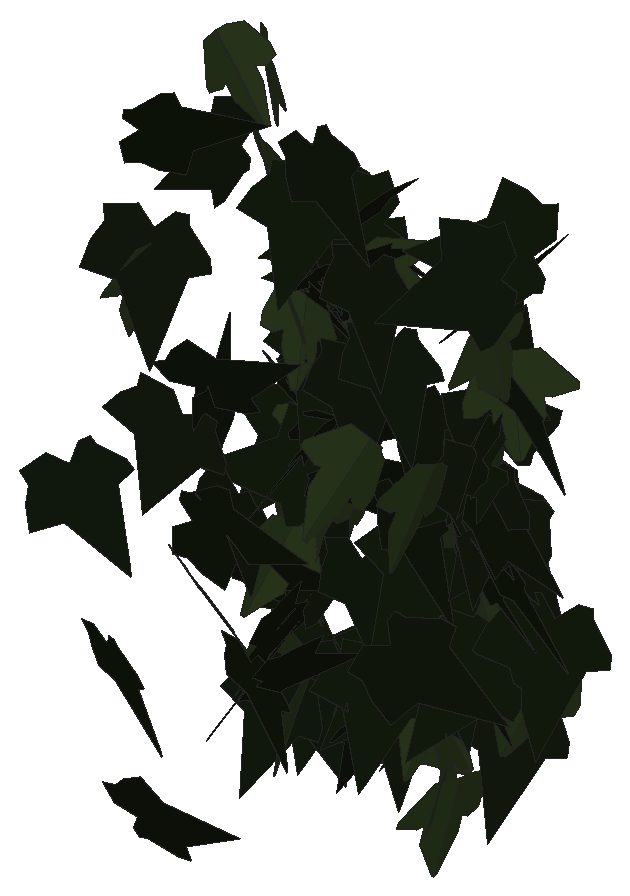
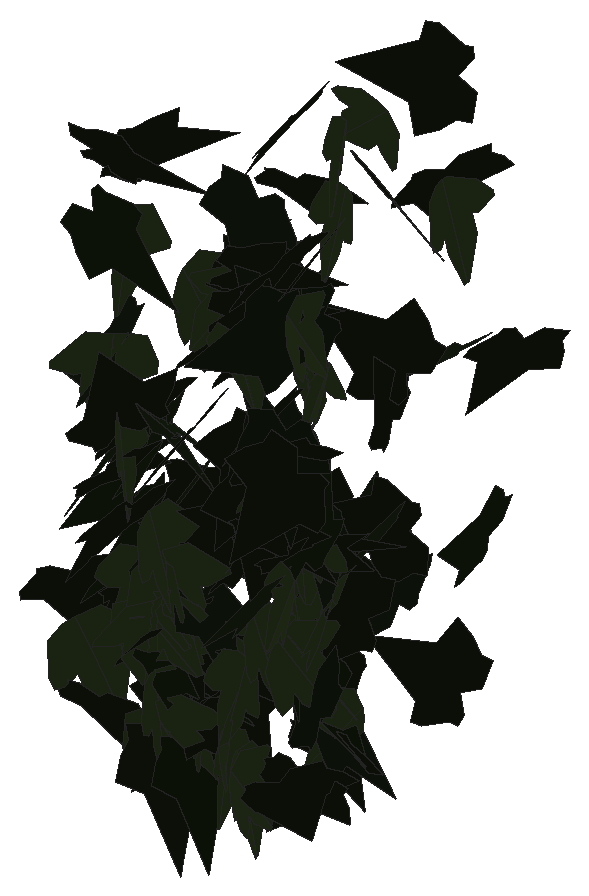
# SketchUp Ruby script. Lengths in inches.
U = 1.inch
M = Sketchup.active_model
def pt(a) = Geom::Point3d.new(a.map { |v| v * U })
def face(e, loops, mat)
  f = e.add_face(loops[0].map { |a| pt(a) })
  loops[1..].each { |l| e.add_face(l.map { |a| pt(a) }).erase! }
  f.material = f.back_material = mat if mat
  f
end
# faces: each face lists its corners as indices into pts; further lists are holes
def faces(e, pts, list, mat = nil) = list.each { |f| face(e, (f[0].is_a?(Array) ? f : [f]).map { |l| l.map { |i| pts[i] } }, mat) }
# xy, xz, yz: faces in a plane at the given z, y or x. An outline is a flat list of corners, or four numbers for a rectangle; further outlines are holes
def ring(l) = l.size == 4 ? [[l[0], l[1]], [l[2], l[1]], [l[2], l[3]], [l[0], l[3]]] : l.each_slice(2).to_a
def flat(e, list, mat, &to3) = list.each { |f| face(e, (f[0].is_a?(Array) ? f : [f]).map { |l| ring(l).map { |u, v| to3.(u, v) } }, mat) }
def xy(e, z, list, mat = nil) = flat(e, list, mat) { |x, y| [x, y, z] }
def xz(e, y, list, mat = nil) = flat(e, list, mat) { |x, z| [x, y, z] }
def yz(e, x, list, mat = nil) = flat(e, list, mat) { |y, z| [x, y, z] }
def lines(e, pts, list) = list.each { |a, b| e.add_line(pt(pts[a]), pt(pts[b])) }
# prism: a flat outline (further loops are holes) pulled along v
def prism(e, loops, v, mat = nil)
  f = face(e, loops, mat); d = Geom::Vector3d.new(v.map { |x| x * U })
  f.pushpull(f.normal.samedirection?(d) ? d.length : -d.length)
end
def box(e, o, s, mat = nil) = prism(e, [[o, [o[0] + s[0], o[1], o[2]], [o[0] + s[0], o[1] + s[1], o[2]], [o[0], o[1] + s[1], o[2]]]], [0, 0, s[2]], mat)
def at(x, y, z, deg = 0) = Geom::Transformation.translation(pt([x, y, z])) * Geom::Transformation.rotation(ORIGIN, Z_AXIS, deg.degrees)
def axes(o, x, y, z) = Geom::Transformation.new([*x, 0, *y, 0, *z, 0, *pt(o).to_a, 1])
def part(name) = M.definitions.add(name)
# library, detail: a bought-in or finely detailed component or shape, given as its bounding box
def library(name, o, s) = part(name).tap { |d| box(d.entities, o, s) }
def detail(e, o, s) = box(e.add_group.entities, o, s)
def put(e, d, t, mat = nil) = e.add_instance(d, t).tap { |i| i.material = mat if mat }
def group(e, t, mat = nil) = e.add_group.tap { |g| g.transformation = t; g.material = mat if mat }.entities
root = M.entities
M.materials.add("efeu1").color = [18, 25, 13]
M.materials.add("efeu2").color = [43, 57, 29]
c1 = part("ivyleaf_9")
p = [[1.54,2.16,1.25],[1.36,2.04,1.19],[-0.21,0.99,0.68],[-0.71,1.11,0.82],[-0.85,0.86,0.67],[-0.8,0.17,0.21],
  [-0.9,-0.01,0.1],[-0.67,-0.16,-0.02],[-0.08,-0.08,-0.05],[-0.03,-0.6,-0.4],[0.65,-0.88,-0.66],[0.83,-0.6,-0.49],
  [1.29,-0.42,-0.43],[1.8125,-0.07,-0.26],[1.21,0.44,0.15]]
faces(c1.entities,p,[[0,1,2,3,4,5,6,7,8,9,10,11,12,13,14]],"efeu1")
c2 = part("ivyleaf_10")
p = [[0,0.5,-0.03],[-0.0625,2.02,-0.43],[-0.19,2.01,-0.46],[-0.54,1.05,-0.29],[-0.52,0.625,-0.18],[-0.83,0.76,-0.28],
  [-1.16,0.64,-0.33],[-1.15,0.33,-0.24],[-0.77,-0.39,0.02],[-0.3,-0.51,0.16],[0.04,-0.48,0.23],[-0.02,2.01,-0.4375],
  [-0.06,2.01,-0.43],[0.04,-0.49,0.23],[0.67,-0.49,0.14],[1.38,0.36,-0.2],[1.375,0.51,-0.24],[0.81,0.65,-0.19],
  [0.62,0.59,-0.15],[0.6,1.09,-0.28],[0.5,1.23,-0.31]]
faces(c2.entities,p,[[0,1,2,3,4,5,6,7,8,9,10],[11,12,0,13,14,15,16,17,18,19,20]],"efeu2")
put(root,c1,axes([7.24,223.58,236.84],[0.37427,-0.2409,-0.10953],[0.09006,-0.06455,0.43891],[-0.2693,-0.3564,-0.00546]))
put(root,c2,axes([7.36,223.84,236.4375],[-0.32136,0.30247,-0.09976],[0.06352,-0.07665,-0.4411],[-0.33676,-0.30309,0.01199]))
put(root,c1,axes([7.35,223.68,237.92],[0.27793,0.32979,0.12409],[0.06108,0.10703,-0.43453],[-0.37381,0.26269,0.02126]))
put(root,c1,axes([7.12,223.52,234.79],[0.11111,-0.2186,0.37621],[0.18138,-0.3205,-0.25111],[0.41889,0.19676,0.00894]))
put(root,c1,axes([7.56,222.75,234.28],[-0.29523,0.23042,-0.25771],[0.14245,-0.2208,-0.36485],[-0.33654,-0.29559,0.07165]))
put(root,c2,axes([7.39,223.09,235.83],[-0.18841,0.3982,-0.0157],[0.00906,-0.01281,-0.45212],[-0.43027,-0.17464,-0.00264]))
put(root,c2,axes([7.46,222.55,234.17],[0.05435,0.1028,0.43646],[-0.12157,0.41104,-0.09067],[-0.45053,-0.09851,0.07712]))
put(root,c1,axes([7.55,223.45,236.71],[-0.32967,-0.3444,0.15068],[-0.05475,-0.1543,-0.47244],[0.37191,-0.328,0.06403]))
put(root,c1,axes([7.44,223.79,233.88],[-0.23188,-0.43865,-0.06175],[0.01831,0.06015,-0.49603],[0.4426,-0.2323,-0.01183]))
put(root,c2,axes([7.55,223.49,235.4],[-0.01446,-0.42559,0.26203],[-0.01458,-0.26167,-0.42581],[0.49958,-0.01995,-0.00484]))
put(root,c1,axes([7.8,221.77,240.93],[-0.40723,0.20452,0.07511],[-0.06788,0.03559,-0.44612],[-0.2242,-0.38227,-0.00135]))
put(root,c1,axes([7.36,219.5,237.84],[0.015,-0.31293,-0.31392],[0.03892,0.30179,-0.32366],[0.46794,-0.01507,0.03698]))
put(root,c2,axes([7.59,220.52,240.05],[0.03065,-0.49801,0.0324],[0.00164,-0.03236,-0.49895],[0.49906,0.0307,-0.00035]))
put(root,c1,axes([7.73,223.78,237.16],[-0.43087,-0.17183,0.02401],[-0.02319,-0.00852,-0.45176],[0.1858,-0.39953,-0.0007]))
put(root,c2,axes([7.68,222.45,241.68],[-0.32271,0.29985,0.10416],[-0.10724,0.04183,-0.4383],[-0.32415,-0.31235,0.0413]))
put(root,c1,axes([7.41,221.6875,235.39],[0.38957,-0.18257,-0.16698],[0.15944,-0.06377,0.42035],[-0.20862,-0.38965,0.00945]))
put(root,c1,axes([7.8,222.75,234.79],[-0.23411,0.322,-0.20421],[0.08926,-0.18042,-0.40258],[-0.39741,-0.2302,0.02988]))
put(root,c2,axes([7.61,223.28,239.59],[0.12695,-0.35049,0.23844],[0.08191,-0.21638,-0.38445],[0.44484,0.13987,0.00274]))
put(root,c1,axes([7.78,223.3,238.13],[0.00225,0.43462,-0.01872],[-0.00118,-0.018,-0.45201],[-0.46979,0.00212,0.00104]))
put(root,c1,axes([7.43,222.25,236.3],[0.0694,-0.39192,0.18456],[0.0824,-0.1662,-0.41048],[0.45728,0.08943,0.04596]))
put(root,c1,axes([8.01,222.94,236.51],[-0.3298,0.04514,0.31875],[-0.3287,-0.124,-0.29639],[0.06241,-0.4145,0.12338]))
put(root,c2,axes([7.6,223.21,236.81],[0.46694,0.03975,0.02779],[0.02546,0.03467,-0.45029],[-0.04503,0.43179,0.0336]))
put(root,c1,axes([7.74,222.7,233.91],[-0.42643,-0.11545,-0.14708],[0.14318,0.05035,-0.42769],[0.13555,-0.41637,-0.01094]))
put(root,c2,axes([7.47,222.06,241.88],[-0.32691,-0.00389,-0.32488],[0.29934,-0.20406,-0.27666],[-0.15569,-0.38415,0.15025]))
put(root,c1,axes([7.5,223.36,233.78],[-0.1878,-0.22057,-0.34546],[0.28115,0.21169,-0.28792],[0.32619,-0.30945,0.04927]))
put(root,c1,axes([7.75,221.4,237.55],[-0.00302,-0.21042,0.39594],[0.15023,0.36029,0.20816],[-0.44512,0.12303,0.06757]))
put(root,c1,axes([7.91,222.47,236.67],[-0.07128,0.40881,0.13852],[-0.01709,0.13235,-0.43064],[-0.46405,-0.06767,-0.00542]))
put(root,c1,axes([7.48,220,235.46],[0.27283,-0.33635,0.11522],[0.06414,-0.09393,-0.43739],[0.37704,0.25936,-0.00897]))
put(root,c2,axes([7.8,223.71,235.7],[0.03527,-0.42599,0.08507],[0.01902,-0.08066,-0.44418],[0.46809,0.03538,0.01164]))
put(root,c1,axes([7.4,221.59,236.27],[0.20707,0.03161,-0.40475],[0.31781,0.27329,0.17385],[0.27718,-0.33696,0.10303]))
put(root,c1,axes([7.68,220.49,240.39],[-0.11012,-0.47615,-0.10561],[0.013,0.10537,-0.4886],[0.48755,-0.11035,-0.01082]))
put(root,c1,axes([8.09,223,235.34],[-0.398,0.2145,0.08953],[-0.08088,0.04246,-0.44345],[-0.23615,-0.37605,0.001]))
put(root,c2,axes([7.75,222.72,238.62],[-0.29857,0.33089,-0.05983],[0.03775,-0.04576,-0.44842],[-0.36075,-0.27865,0.00259]))
put(root,c2,axes([7.83,222.57,235.77],[0.1551,0.30588,-0.28489],[-0.13785,-0.24257,-0.35129],[-0.42149,0.19189,0.01006]))
put(root,c1,axes([7.4,222.35,235.47],[0.25502,-0.08858,0.36861],[0.37425,-0.07933,-0.26073],[0.12494,0.41843,0.0286]))
put(root,c2,axes([7.87,222.23,240.65],[-0.39979,0.22056,0.06194],[-0.05517,0.03062,-0.44814],[-0.24049,-0.37369,-0.00016]))
put(root,c1,axes([7.58,223.86,236.39],[0.3108,-0.31463,-0.08959],[-0.00923,0.10757,-0.43826],[0.35218,0.28047,0.06758]))
put(root,c2,axes([7.79,223.53,237.76],[-0.04218,0.42973,-0.05723],[-0.00017,-0.05527,-0.44873],[-0.4679,-0.03872,0.00532]))
put(root,c1,axes([7.84,223.48,237.88],[-0.24948,-0.36844,-0.01136],[0.00513,0.00991,-0.45226],[0.39805,-0.23104,-0.00129]))
put(root,c1,axes([7.72,220.89,237.97],[-0.18046,-0.42997,0.18045],[0.11887,-0.22952,-0.42801],[0.45089,-0.11157,0.18506]))
put(root,c2,axes([7.86,223.99,233.84],[0.11769,-0.34318,0.25385],[0.08691,-0.23051,-0.37442],[0.44644,0.13535,0.00597]))
put(root,c1,axes([7.9,222.03,234.78],[0.0902,0.24019,0.36705],[0.15191,0.32406,-0.26398],[-0.43532,0.16285,-0.01606]))
put(root,c1,axes([7.625,220.43,241.65],[0.17402,0.2237,-0.34995],[0.15382,0.30756,0.28357],[0.40837,-0.21117,0.04231]))
put(root,c2,axes([8.06,222.93,236.18],[0.25243,-0.3119,-0.20089],[-0.10324,0.16935,-0.40468],[0.38253,0.25152,0.02336]))
put(root,c2,axes([8.02,223.75,233.82],[0.12082,-0.48391,-0.03513],[-0.00062,0.03605,-0.4987],[0.48518,0.12055,0.00811]))
put(root,c2,axes([7.79,224.4,234.52],[0.06042,-0.17406,0.4105],[0.31712,-0.27622,-0.16996],[0.34131,0.28746,0.08525]))
put(root,c1,axes([7.66,221.31,238.17],[0.0865,-0.13267,0.42272],[0.45455,-0.0484,-0.10267],[0.08136,0.41144,0.12423]))
put(root,c1,axes([7.78,223.3125,239.43],[0.42696,-0.07853,0.17015],[0.17861,-0.00561,-0.41839],[0.08071,0.42782,0.02575]))
put(root,c1,axes([8.16,223.08,237.15],[0.27483,0.33066,-0.12793],[-0.07628,-0.10085,-0.4339],[-0.37331,0.26404,-0.00552]))
put(root,c2,axes([8.13,222.39,234.06],[0.20988,-0.37631,0.10321],[0.03954,-0.09276,-0.44035],[0.41845,0.19751,-0.01016]))
put(root,c2,axes([8.04,222.5625,238.71],[0.45478,-0.08414,0.07227],[0.0747,-0.00851,-0.44656],[0.09117,0.4267,0.00535]))
put(root,c1,axes([7.77,220.18,233.43],[0.17525,-0.12796,0.39809],[0.38661,-0.14492,-0.2082],[0.20133,0.38968,0.0533]))
put(root,c1,axes([8,222.46,240.06],[0.22938,-0.36692,-0.10129],[-0.04876,0.08639,-0.4409],[0.40709,0.2171,0.00426]))
put(root,c1,axes([8,222.38,239.22],[0.45822,-0.09587,-0.00494],[-0.00477,0.00201,-0.45237],[0.10356,0.4243,0.00102]))
put(root,c1,axes([8.15,223.06,240.07],[-0.01314,-0.4924,0.08583],[0.01297,-0.08617,-0.49235],[0.49966,-0.01071,0.01504]))
put(root,c2,axes([8.34,223.46,234.86],[-0.43023,0.17463,0.00638],[-0.00592,0.00278,-0.45235],[-0.18863,-0.3984,-0.00036]))
put(root,c2,axes([8.38,223.54,233.92],[0.04319,-0.38271,-0.21099],[0.02045,0.20509,-0.39848],[0.46736,0.0264,0.03693]))
put(root,c1,axes([8.2,223.18,238.1],[0.08535,-0.42674,0.03079],[0.00045,-0.03003,-0.45132],[0.46198,0.07887,-0.00525]))
put(root,c1,axes([8.65,222.35,237.65],[-0.13206,0.41668,-0.02647],[0.00663,-0.02473,-0.45162],[-0.45081,-0.12243,0.00111]))
put(root,c2,axes([8.45,223.28,239.05],[0.46578,-0.05548,-0.01255],[-0.01233,0.00586,-0.4522],[0.06007,0.43141,0.00453]))
put(root,c1,axes([8.77,222.96,239.8],[-0.33348,-0.12842,0.28931],[-0.27281,-0.11682,-0.34769],[0.18728,-0.39886,0.00868]))
put(root,c1,axes([8.79,223.05,239.25],[-0.28513,-0.08425,0.34871],[-0.3257,-0.15017,-0.28619],[0.18258,-0.39947,0.03404]))
put(root,c1,axes([8.84,222.32,239.61],[0.09514,0.42321,-0.05052],[-0.08205,-0.0332,-0.44411],[-0.45269,0.09496,0.06988]))
put(root,c1,axes([8.67,221.95,240.58],[-0.33889,-0.27027,-0.13843],[0.17107,0.01548,-0.42103],[0.27677,-0.3405,0.09074]))
put(root,c1,axes([8.95,223.51,233.51],[-0.07791,0.42875,0.01459],[0.00265,0.01464,-0.45214],[-0.46329,-0.07201,-0.00504]))
put(root,c1,axes([9,222.77,234.05],[-0.07824,0.35528,-0.24994],[0.05215,-0.23542,-0.37709],[-0.46029,-0.08707,-0.00024]))
put(root,c1,axes([9.03,222.27,240.3],[0.06921,0.41652,0.11217],[-0.03938,0.11391,-0.43496],[-0.463,0.05257,0.05376]))
put(root,c1,axes([8.88,222.26,237.1],[0.31532,0.32232,0.00991],[0.0061,0.00774,-0.45229],[-0.3482,0.29202,0.00105]))
put(root,c1,axes([9.11,223.04,234.52],[-0.39555,-0.21944,0.08659],[-0.06459,-0.06196,-0.44345],[0.24511,-0.37045,0.02287]))
put(root,c1,axes([9.18,223.75,233.69],[-0.07636,0.49393,-0.01421],[0.00261,-0.01398,-0.4998],[-0.49413,-0.0764,-0.00044]))
put(root,c2,axes([8.89,222.71,239.4],[0.17982,0.27963,0.30018],[0.09937,0.2776,-0.3349],[-0.4225,0.1843,0.04899]))
put(root,c1,axes([9.25,222.93,235.37],[-0.16193,0.40305,-0.06816],[0.02479,-0.06139,-0.44724],[-0.44031,-0.15168,-0.00011]))
put(root,c1,axes([8.9,222.53,235.88],[0.08792,-0.42731,0.00021],[-0.00018,-0.00024,-0.4524],[0.4615,0.08141,-0.00021]))
put(root,c1,axes([8.88,221.75,241.26],[0.2056,-0.37235,-0.12454],[-0.02612,0.12172,-0.4336],[0.42161,0.18912,0.03387]))
put(root,c1,axes([8.875,220.69,235.43],[0.18382,-0.37218,0.15334],[0.07343,-0.13102,-0.42556],[0.42606,0.18315,0.00718]))
put(root,c2,axes([9.27,223.7,234.0625],[0.39775,0.15781,-0.25863],[-0.24225,-0.09067,-0.42789],[-0.18195,0.4657,0.00433]))
put(root,c1,axes([9.03,222.98,234.16],[0.00883,-0.43298,0.04274],[0.00218,-0.04107,-0.45037],[0.46971,0.00833,0.00129]))
put(root,c1,axes([9.04,222.3,238.38],[-0.00737,-0.43401,0.02964],[0.00314,-0.02855,-0.45141],[0.46973,-0.00662,0.00348]))
put(root,c1,axes([9.15,222.6,234.61],[-0.30956,-0.29937,-0.13738],[0.1393,0.05802,-0.42782],[0.32478,-0.31022,0.05256]))
put(root,c1,axes([9.08,223.23,234.16],[0.41106,0.21058,0.00462],[0.00054,0.00827,-0.45232],[-0.22747,0.38054,0.00727]))
put(root,c2,axes([9.14,222.83,234.81],[0.28561,0.31863,0.13862],[0.02167,0.15341,-0.42282],[-0.37238,0.25331,0.08171]))
put(root,c2,axes([9.3,223.69,234.39],[0.06413,-0.4862,-0.09745],[-0.00478,0.09765,-0.49035],[0.49585,0.06383,0.00788]))
put(root,c2,axes([9.18,223.15,233.86],[-0.25453,-0.34082,-0.26279],[0.19518,0.18069,-0.42339],[0.38356,-0.31811,0.04106]))
put(root,c1,axes([9.14,220.61,235.4],[0.24173,0.21025,0.32042],[0.18207,0.2635,-0.31438],[-0.35934,0.27494,0.05627]))
put(root,c2,axes([9.41,223.43,235.82],[-0.28727,-0.38682,0.13358],[-0.0208,-0.1492,-0.47677],[0.40871,-0.27948,0.06963]))
put(root,c2,axes([9.32,223.21,233.74],[-0.41049,0.20997,-0.027],[0.02778,-0.00712,-0.45155],[-0.2268,-0.3809,-0.00644]))
put(root,c1,axes([9.2,222.28,239.66],[0.04449,-0.433,-0.00651],[-0.00845,0.00554,-0.45229],[0.46761,0.04129,-0.00755]))
put(root,c1,axes([9.63,223.21,234.73],[-0.34698,0.27641,-0.23065],[0.05369,-0.27703,-0.41276],[-0.35598,-0.31121,0.16256]))
put(root,c1,axes([9.24,222.59,238.625],[0.02375,-0.43213,-0.04655],[0.0476,0.0468,-0.44743],[0.46678,0.01722,0.04799]))
put(root,c2,axes([9.41,223.01,234.53],[-0.15339,-0.44466,-0.16957],[0.11186,0.13948,-0.46694],[0.46256,-0.18118,0.05669]))
put(root,c2,axes([9.52,223.47,236.33],[0.04445,-0.49708,0.03056],[-0.00088,-0.03076,-0.49905],[0.49802,0.04431,-0.00361]))
put(root,c2,axes([9.59,223.54,235.29],[0.42335,0.12095,-0.23695],[-0.22415,-0.07768,-0.44014],[-0.14328,0.47889,-0.01155]))
put(root,c2,axes([9.49,223,234.25],[-0.11014,-0.34764,0.2504],[0.09641,-0.25979,-0.35079],[0.44641,-0.02966,0.13754]))
put(root,c1,axes([9.3125,223.09,237.59],[0.26218,-0.40407,-0.13411],[-0.03949,0.13374,-0.48016],[0.42391,0.26237,0.03822]))
put(root,c1,axes([9.66,222.91,236.13],[-0.38768,-0.31571,0.00534],[-0.00392,-0.00364,-0.49997],[0.31573,-0.3877,0.00035]))
put(root,c2,axes([9.53,223.6,235.29],[0.17762,0.46733,-0.00728],[-0.01244,-0.00305,-0.49984],[-0.46722,0.17774,0.01055]))
put(root,c1,axes([9.46,223.35,235.04],[0.01288,-0.49691,-0.05401],[0.04472,0.05496,-0.49495],[0.49783,0.00792,0.04586]))
put(root,c2,axes([9.71,223.46,235.72],[-0.49115,0.00395,-0.09355],[0.09252,-0.0562,-0.48814],[-0.01437,-0.49682,0.05447]))
put(root,c1,axes([9.51,222.51,236.85],[0.25252,-0.42795,-0.05565],[-0.0323,0.04555,-0.49687],[0.43034,0.25453,-0.00464]))
put(root,c1,axes([10.3,222.76,237.53],[-0.40546,0.29247,0.00815],[-0.02446,-0.02001,-0.499],[-0.29155,-0.40505,0.03053]))
put(root,c2,axes([10.08,223.39,237.4],[0.18213,-0.45381,-0.10433],[0.00022,0.11211,-0.48727],[0.46565,0.17744,0.04104]))
put(root,c2,axes([10.09,220.92,238.3],[-0.12612,-0.30084,0.37893],[0.05902,-0.39824,-0.29652],[0.48022,-0.03007,0.13596]))
put(root,c1,axes([10.14,223.35,237.48],[-0.25952,-0.21664,0.3684],[0.28143,0.23774,0.33805],[-0.32163,0.38282,-0.00146]))
put(root,c1,axes([10.375,222.79,237.48],[-0.48447,0.12319,-0.01072],[-0.0179,-0.11275,-0.48679],[-0.12235,-0.47129,0.11366]))
put(root,c1,axes([9.91,223.48,236.52],[0.18302,-0.39617,-0.24404],[-0.01548,0.25691,-0.42867],[0.46504,0.16446,0.08178]))
put(root,c1,axes([9.94,223.08,236.15],[0.42615,-0.23893,-0.10633],[-0.09014,0.05663,-0.48854],[0.24549,0.43555,0.0052]))
put(root,c1,axes([10.14,223.71,234.02],[-0.37795,-0.24606,-0.21588],[0.22968,0.0356,-0.4427],[0.23324,-0.4338,0.08612]))
put(root,c1,axes([10.29,222.875,235.12],[-0.30956,-0.37379,0.12022],[-0.05675,-0.10888,-0.48469],[0.38852,-0.31373,0.02498]))
put(root,c1,axes([10.01,222.83,237.11],[0.34121,-0.35604,-0.08254],[-0.06463,0.05236,-0.49303],[0.35972,0.34712,-0.01029]))
put(root,c1,axes([9.96,222.82,235.03],[0.22833,-0.36348,0.25641],[0.18389,-0.1853,-0.42644],[0.40503,0.28904,0.04906]))
put(root,c1,axes([10.34,223.33,236.79],[-0.22917,-0.39662,0.20044],[-0.01363,-0.21914,-0.44921],[0.44418,-0.21135,0.08963]))
put(root,c2,axes([10.32,223.3,238.35],[0.32959,0.37157,0.05753],[-0.03008,0.10231,-0.4885],[-0.37479,0.31854,0.08979]))
put(root,c2,axes([10.57,223.49,234.58],[-0.27241,-0.36552,0.2054],[-0.12323,-0.16432,-0.45586],[0.40075,-0.29899,-0.00056]))
put(root,c2,axes([10.51,221.87,234.19],[0.22982,-0.40373,-0.18489],[-0.05449,0.18098,-0.4629],[0.4407,0.23292,0.03919]))
put(root,c1,axes([10.32,222.82,237.3],[-0.00876,-0.49603,0.0623],[-0.01397,-0.06204,-0.49594],[0.49973,-0.01043,-0.01277]))
put(root,c1,axes([10.125,221.5625,235.7],[0.04813,-0.04956,-0.4952],[0.29863,0.40087,-0.01109],[0.39812,-0.2947,0.06819]))
put(root,c1,axes([10.73,223.07,239.87],[-0.3144,0.34323,-0.18261],[0.01053,-0.22725,-0.44525],[-0.38864,-0.28381,0.13567]))
put(root,c2,axes([10.62,221.91,233.9375],[-0.05991,-0.49198,0.06608],[0.01239,-0.06802,-0.4952],[0.49624,-0.0577,0.02034]))
put(root,c1,axes([10.32,223.27,238.34],[0.28648,-0.3899,0.12612],[0.07568,-0.1009,-0.48383],[0.40274,0.2963,0.0012]))
put(root,c1,axes([10.49,222.65,237.13],[0.34673,-0.23297,-0.27478],[-0.1734,0.22637,-0.41072],[0.31577,0.38011,0.07618]))
put(root,c1,axes([11.1,222.59,240.4],[-0.37178,0.12837,0.3087],[-0.31629,0.01454,-0.38697],[-0.10832,-0.48302,0.07039]))
put(root,c2,axes([10.76,222.39,239.4],[-0.01755,-0.47765,-0.14677],[0.07983,0.1423,-0.47263],[0.49327,-0.04002,0.07127]))
put(root,c1,axes([10.51,222.77,236.43],[0.38986,-0.31295,0.00846],[0.00703,-0.00476,-0.49993],[0.31298,0.38993,0.00069]))
put(root,c2,axes([10.8,221.2,238.11],[0.03474,-0.45285,0.2091],[0.04741,-0.20566,-0.45327],[0.49653,0.05132,0.02865]))
put(root,c1,axes([10.98,222.19,240.22],[-0.26589,-0.20505,0.37048],[-0.26456,-0.26113,-0.33439],[0.33062,-0.37385,0.03037]))
put(root,c1,axes([10.73,223.49,235.37],[-0.23666,-0.41843,-0.1375],[0.05565,0.12644,-0.48054],[0.43692,-0.24275,-0.01328]))
